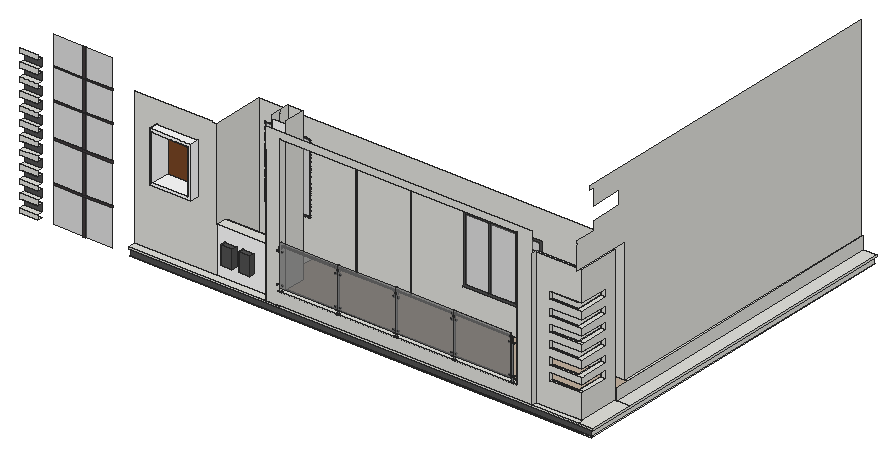
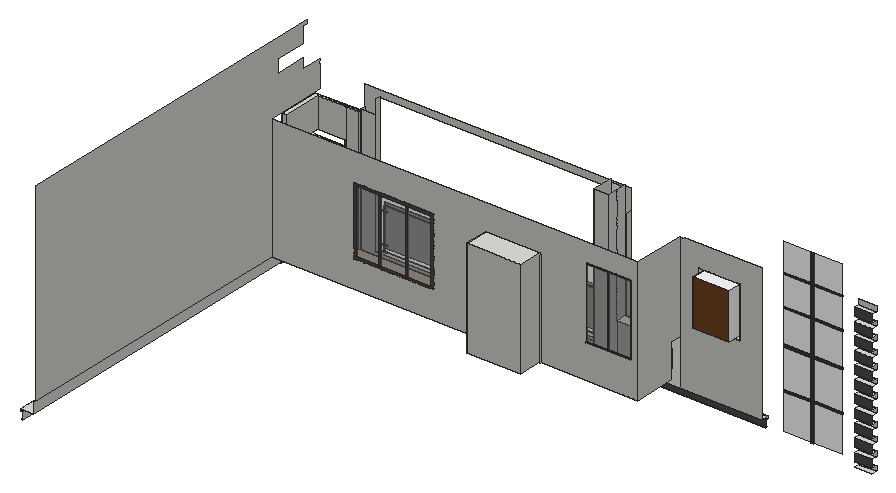
# SketchUp Ruby script. Lengths in inches.
U = 1.inch
M = Sketchup.active_model
def pt(a) = Geom::Point3d.new(a.map { |v| v * U })
def face(e, loops, mat)
  f = e.add_face(loops[0].map { |a| pt(a) })
  loops[1..].each { |l| e.add_face(l.map { |a| pt(a) }).erase! }
  f.material = f.back_material = mat if mat
  f
end
# faces: each face lists its corners as indices into pts; further lists are holes
def faces(e, pts, list, mat = nil) = list.each { |f| face(e, (f[0].is_a?(Array) ? f : [f]).map { |l| l.map { |i| pts[i] } }, mat) }
# xy, xz, yz: faces in a plane at the given z, y or x. An outline is a flat list of corners, or four numbers for a rectangle; further outlines are holes
def ring(l) = l.size == 4 ? [[l[0], l[1]], [l[2], l[1]], [l[2], l[3]], [l[0], l[3]]] : l.each_slice(2).to_a
def flat(e, list, mat, &to3) = list.each { |f| face(e, (f[0].is_a?(Array) ? f : [f]).map { |l| ring(l).map { |u, v| to3.(u, v) } }, mat) }
def xy(e, z, list, mat = nil) = flat(e, list, mat) { |x, y| [x, y, z] }
def xz(e, y, list, mat = nil) = flat(e, list, mat) { |x, z| [x, y, z] }
def yz(e, x, list, mat = nil) = flat(e, list, mat) { |y, z| [x, y, z] }
def lines(e, pts, list) = list.each { |a, b| e.add_line(pt(pts[a]), pt(pts[b])) }
# prism: a flat outline (further loops are holes) pulled along v
def prism(e, loops, v, mat = nil)
  f = face(e, loops, mat); d = Geom::Vector3d.new(v.map { |x| x * U })
  f.pushpull(f.normal.samedirection?(d) ? d.length : -d.length)
end
def box(e, o, s, mat = nil) = prism(e, [[o, [o[0] + s[0], o[1], o[2]], [o[0] + s[0], o[1] + s[1], o[2]], [o[0], o[1] + s[1], o[2]]]], [0, 0, s[2]], mat)
def at(x, y, z, deg = 0) = Geom::Transformation.translation(pt([x, y, z])) * Geom::Transformation.rotation(ORIGIN, Z_AXIS, deg.degrees)
def axes(o, x, y, z) = Geom::Transformation.new([*x, 0, *y, 0, *z, 0, *pt(o).to_a, 1])
def part(name) = M.definitions.add(name)
# library, detail: a bought-in or finely detailed component or shape, given as its bounding box
def library(name, o, s) = part(name).tap { |d| box(d.entities, o, s) }
def detail(e, o, s) = box(e.add_group.entities, o, s)
def put(e, d, t, mat = nil) = e.add_instance(d, t).tap { |i| i.material = mat if mat }
def group(e, t, mat = nil) = e.add_group.tap { |g| g.transformation = t; g.material = mat if mat }.entities
root = M.entities
M.materials.add("[0128_White]").color = [255, 255, 255]
M.materials.add("[0135_DarkGray]").color = [81, 81, 81]
M.materials.add("[Asphalt New]").color = [67, 60, 62]
M.materials.add("[Granite Brown]").color = [113, 117, 119]
M.materials.add("[Granite Light Gray]").color = [139, 143, 145]
M.materials.add("[Stone Brushed Khaki]").color = [166, 166, 164]
M.materials.add("[Tile Large Brown]").color = [195, 178, 159]
M.materials.add("[Translucent Glass Gray]").color = [128, 128, 128]
M.materials["[Translucent Glass Gray]"].alpha = 0.5
M.materials.add("[Wood Veneer 01]").color = [120, 70, 37]
M.materials.add("archibd _ glass railing _ 8mm glass").color = [128, 128, 128]
M.materials["archibd _ glass railing _ 8mm glass"].alpha = 0.5
c1 = part("DOOR12")
g1 = group(c1.entities,at(114.73,28.14,-0.51))
g2 = group(g1,at(0,0,0))
box(g2,[0,0,0],[36,0.5,77.7])
c2 = part("archibd _ glass railing _  tophandrail")
box(c2.entities,[0,0,0],[47.24,2.95,0.98],"[Stone Brushed Khaki]")
c3 = part("archibd _ glass railing _  8 mm Glass")
box(c3.entities,[0.2,-0.31,2.95],[46.85,0.31,44.29],"archibd _ glass railing _ 8mm glass")
p = [[47.05,0,2.95],[47.24,0,2.95],[0.2,0,2.95],[0,0,2.95]]
lines(c3.entities,p,[[0,1],[2,3]])
c4 = part("archibd _ glass railing _  post 1")
box(c4.entities,[-0.04,0,0],[0.47,2.95,41.34],"[Granite Light Gray]")
c5 = part("archibd _ glass railing _ joint plate")
box(c5.entities,[0.98,0.98,-0.31],[2.96,4.93,0.31],"[Granite Light Gray]")
c6 = part("archibd _ glass railing _  post knob")
prism(c6.entities,[[[0.43,1.22,0],[0.43,1.97,0],[0.43,1.97,2.95],[0.43,0,2.95],[0.43,0,0],[0.43,0.75,0],[0.43,0.75,0.98],[0.43,1.22,0.98]]],[-0.47,0,0],"[Granite Light Gray]")
c7 = part("archibd _ glass railing _ serew")
xy(c7.entities,0,[[0.16,0,0,0.27,0.16,0.55,0.47,0.55,0.63,0.27,0.47,0]],"[Granite Brown]")
xy(c7.entities,0.2,[[0.16,0,0.47,0,0.63,0.27,0.47,0.55,0.16,0.55,0,0.27]],"[Granite Brown]")
xz(c7.entities,0,[[0.16,0,0.47,0.2]],"[Granite Brown]")
xz(c7.entities,0.55,[[0.16,0,0.47,0.2]],"[Granite Brown]")
p = [[0,0.27,0],[0.16,0,0],[0.16,0,0.2],[0,0.27,0.2],[0.47,0,0],[0.63,0.27,0],
  [0.63,0.27,0.2],[0.47,0,0.2],[0.16,0.55,0],[0.16,0.55,0.2],[0.47,0.55,0],[0.47,0.55,0.2]]
faces(c7.entities,p,[[0,1,2,3],[4,5,6,7],[8,0,3,9],[5,10,11,6]],"[Granite Brown]")
c8 = part("archibd _ glass railing _  knob 1")
xy(c8.entities,-0.2,[[1.26,-0.47,1.97,-0.24],[1.26,0.08,1.26,2.76,0,2.76,0,3.46,1.97,3.46,1.97,0.08]],"[Granite Light Gray]")
xy(c8.entities,-0.12,[[1.34,-0.24,1.89,0.08]],"[Granite Brown]")
xy(c8.entities,0.43,[[1.34,-0.24,1.89,0.08]],"[Granite Brown]")
xy(c8.entities,0.51,[[1.26,-0.47,1.97,-0.24],[1.26,0.08,1.97,0.08,1.97,3.46,0,3.46,0,2.76,1.26,2.76]],"[Granite Light Gray]")
xz(c8.entities,-0.47,[[1.26,-0.2,1.97,0.51]],"[Granite Light Gray]")
xz(c8.entities,-0.24,[[[1.26,-0.2,1.97,0.51],[1.34,-0.12,1.89,0.43]],[1.34,-0.12,1.89,0.43]],"[Granite Light Gray]")
xz(c8.entities,0.08,[[[1.26,-0.2,1.97,0.51],[1.34,-0.12,1.89,0.43]],[1.34,-0.12,1.89,0.43]],"[Granite Light Gray]")
xz(c8.entities,2.76,[[0,-0.2,1.26,0.51]],"[Granite Light Gray]")
xz(c8.entities,3.46,[[0,-0.2,1.97,0.51]],"[Granite Light Gray]")
yz(c8.entities,0,[[2.76,-0.2,3.46,0.51]],"[Granite Light Gray]")
yz(c8.entities,1.26,[[-0.47,-0.2,-0.24,0.51],[0.08,-0.2,2.76,0.51]],"[Granite Light Gray]")
yz(c8.entities,1.34,[[-0.24,-0.12,0.08,0.43]],"[Granite Brown]")
yz(c8.entities,1.89,[[-0.24,-0.12,0.08,0.43]],"[Granite Brown]")
yz(c8.entities,1.97,[[-0.47,-0.2,-0.24,0.51],[0.08,-0.2,3.46,0.51]],"[Granite Light Gray]")
c9 = part("archibd _ glass railing _  knob 2")
put(c9.entities,c8,at(2.4,0,0))
put(c9.entities,c8,axes([1.93,0,0],[-1,0,0],[0,1,0],[0,0,1]))
c10 = part("archibd _ glass railing _  post")
put(c10.entities,c4,at(1.28,0.98,0.31))
put(c10.entities,c5,at(-0.98,-0.98,0.31))
put(c10.entities,c6,at(0.49,2.66,40.67,-90))
put(c10.entities,c7,at(0.31,4.02,0.31))
put(c10.entities,c7,at(0.31,0.36,0.31))
put(c10.entities,c7,at(2.01,4.02,0.31))
put(c10.entities,c7,at(2.01,0.36,0.31))
put(c10.entities,c9,at(-0.6875,-0.75,6.42))
put(c10.entities,c9,at(-0.6875,-0.65,38.1875))
c11 = part("archibd _ modern glass railing _ 1")
put(c11.entities,c2,at(2.2,2.2,43.62))
put(c11.entities,c3,at(2.2,0.65,0.31))
put(c11.entities,c10,at(0.73,1.22,0))
put(c11.entities,c10,at(47.97,1.22,0))
c12 = part("Archibd+_+Glass+Railing+_+Modern+Glass+Railing+_+1")
put(c12.entities,c11,at(11.52,12.04,0))
put(c12.entities,c11,at(153.25,12.04,0))
put(c12.entities,c11,at(106.01,12.04,0))
put(c12.entities,c11,at(58.76,12.04,0))
xy(root,324.03,[[532.875,578.55,567.67,588.61]])
xy(root,325.125,[[749.43,575.61,1658.1875,575.61,1658.1875,577.48,1630.5625,577.48,1630.5625,578.42,749.43,578.42],[1630.5625,577.48,1658.1875,577.48,1658.1875,1270.99,1655,1270.99,1655,578.42,1630.5625,578.42]])
xy(root,333.75,[[532.875,578.55,567.67,588.61]])
xy(root,338.38,[[749.43,573.8,749.43,578.42,1630.5625,578.42,1630.5625,577.48,1660.625,577.48,1660.625,573.8],[1630.5625,577.48,1660.625,578.42],[1655,578.42,1660.625,1270.99]])
xy(root,341.71,[[1018.16,573.8,1047.4,584.05]])
xy(root,342.73,[[749.43,573.8,1047.4,573.8,1047.4,584.05,1541.95,584.05,1541.95,588.61,749.43,588.61],[1047.4,573.8,1541.95,584.05],[1541.95,573.8,1634.625,583.86],[1634.625,573.8,1660.625,573.8,1660.625,665.53,1631.1875,665.53,1631.1875,583.86,1634.625,583.86],[1634.625,665.53,1660.625,1270.99]])
xy(root,349.59,[[532.875,578.55,567.67,588.61]])
xy(root,359.32,[[532.875,578.55,567.67,588.61]])
xy(root,365.875,[[910.24,610.34,1018.14,691.875],[1633.375,690.6875,1634.625,690.6875,1634.625,1270.99,1630.5,1270.99,1630.5,691.875,1633.375,691.875]])
xy(root,365.875,[[1047.4,588.61,1621.25,588.61,1621.25,665.53,1634.625,665.53,1634.625,690.6875,1633.375,690.6875,1633.375,691.875,1208.65,691.875,1208.65,739.5,1102.33,739.5,1102.33,691.875,1018.14,691.875,1018.14,628.55,1047.4,628.55]],"[Tile Large Brown]")
xy(root,368.26,[[1047.4,573.8,1512.22,584.05]])
xy(root,370.97,[[927.55,577.92,949.64,588.61],[962.05,577.92,984.14,588.61]],"[0135_DarkGray]")
xy(root,375.15,[[532.875,578.55,567.67,588.61]])
xy(root,384.88,[[532.875,578.55,567.67,588.61]])
xy(root,390.46,[[1568.17,583.86,1631.1875,588.61],[1621.25,588.61,1631.1875,642.95]])
xy(root,400.71,[[532.875,578.55,567.67,588.61]])
xy(root,405.06,[[1568.17,583.86,1631.1875,588.61],[1621.25,588.61,1631.1875,642.95]])
xy(root,406.7,[[927.55,577.92,949.64,588.61],[962.05,577.92,984.14,588.61]],"[0135_DarkGray]")
xy(root,410.44,[[532.875,578.55,567.67,588.61]])
xy(root,418.09,[[1568.17,583.86,1631.1875,583.86,1631.1875,642.95,1621.25,642.95,1621.25,588.61,1568.17,588.61]])
xy(root,426.28,[[532.875,578.55,567.67,588.61]])
xy(root,432.68,[[1568.17,583.86,1631.1875,588.61],[1621.25,588.61,1631.1875,642.95]])
xy(root,432.6875,[[910.24,588.61,1018.14,610.34]])
xy(root,436,[[532.875,578.55,567.67,588.61]])
xy(root,447.78,[[1568.17,583.86,1631.1875,583.86,1631.1875,642.95,1621.25,642.95,1621.25,588.61,1568.17,588.61]])
xy(root,451.84,[[532.875,578.55,567.67,588.61]])
xy(root,461.57,[[532.875,578.55,567.67,588.61]])
xy(root,462.37,[[1568.17,583.86,1631.1875,588.61],[1621.25,588.61,1631.1875,642.95]])
xy(root,467.37,[[792.08,571.8,873.44,588.61]],"[0128_White]")
xy(root,472.64,[[797.35,571.8,868.17,609.98]],"[0128_White]")
xy(root,476.09,[[1568.17,583.86,1631.1875,588.61],[1621.25,588.61,1631.1875,642.95]])
xy(root,477.4,[[532.875,578.55,567.67,588.61]])
xy(root,487.13,[[532.875,578.55,567.67,588.61]])
xy(root,490.68,[[1568.17,583.86,1631.1875,588.61],[1621.25,588.61,1631.1875,642.95]])
xy(root,502.96,[[532.875,578.55,567.67,588.61]])
xy(root,504.09,[[1568.17,583.86,1631.1875,583.86,1631.1875,642.95,1621.25,642.95,1621.25,588.61,1568.17,588.61]])
xy(root,512.69,[[532.875,578.55,567.67,588.61]])
xy(root,518.68,[[1568.17,583.86,1631.1875,588.61],[1621.25,588.61,1631.1875,642.95]])
xy(root,528.53,[[532.875,578.55,567.67,588.61]])
xy(root,533.84,[[1568.17,583.86,1621.25,588.61],[1621.25,583.86,1631.1875,642.95]])
xy(root,538.25,[[532.875,578.55,567.67,588.61]])
xy(root,548.43,[[1568.17,583.86,1621.25,588.61],[1621.25,583.86,1631.1875,642.95]])
xy(root,554.09,[[532.875,578.55,567.67,588.61]])
xy(root,558.75,[[1102.33,691.875,1208.65,739.5]])
xy(root,562.02,[[797.35,571.8,868.17,609.98]],"[0128_White]")
xy(root,563.82,[[532.875,578.55,567.67,588.61]])
xy(root,567.29,[[792.08,571.8,873.44,588.61]],"[0128_White]")
xy(root,579.65,[[532.875,578.55,567.67,588.61]])
xy(root,589.38,[[532.875,578.55,567.67,588.61]])
xy(root,605.21,[[532.875,578.55,567.67,588.61]])
xy(root,607.25,[[1541.95,583.86,1631.1875,583.86,1631.1875,665.53,1621.25,665.53,1621.25,588.61,1541.95,588.61]])
xz(root,571.8,[[[792.08,467.37,873.44,567.29],[797.35,472.64,868.17,562.02]]],"[0128_White]")
xz(root,573.8,[[749.43,338.38,1660.625,338.38,1660.625,342.73,1047.4,342.73,1047.4,341.71,1018.16,341.71,1018.16,342.73,749.43,342.73],[1018.16,341.71,1047.4,342.73],[[1018.16,342.73,1541.95,649.875],[1047.4,368.26,1512.22,637.28]]])
xz(root,575.61,[[658.55,327.45,664.15,398.34],[600.1,398.34,658.55,402.19],[658.55,398.34,664.15,402.19],[664.15,398.34,716.99,402.19],[658.55,402.19,664.15,476.93],
  [600.1,476.93,658.55,481.65],[658.55,476.93,664.15,481.65],[664.15,476.93,716.99,481.65],[658.55,481.65,664.15,545.03],[600.1,545.03,658.55,547.98],
  [658.55,545.03,664.15,547.98],[664.15,545.03,716.99,547.98],[658.55,547.98,664.15,605.5],[600.1,605.5,658.55,607.82],[658.55,605.5,664.15,607.82],
  [664.15,605.5,716.99,607.82],[658.55,607.82,664.15,663.68]],"[Asphalt New]")
xz(root,575.61,[[600.1,327.45,658.55,398.34],[664.15,327.45,716.99,398.34],[600.1,402.19,658.55,476.93],[664.15,402.19,716.99,476.93],[600.1,481.65,658.55,545.03],
  [664.15,481.65,716.99,545.03],[600.1,547.98,658.55,605.5],[664.15,547.98,716.99,605.5],[600.1,607.82,658.55,663.68],[664.15,607.82,716.99,663.68]],"[Translucent Glass Gray]")
xz(root,577.92,[[927.55,370.97,949.64,406.7],[962.05,370.97,984.14,406.7]],"[0135_DarkGray]")
xz(root,578.42,[[749.43,325.125,1655,338.38]],"[0135_DarkGray]")
xz(root,578.55,[[532.875,324.03,567.67,333.75],[532.875,349.59,567.67,359.32],[532.875,375.15,567.67,384.88],[532.875,400.71,567.67,410.44],[532.875,426.28,567.67,436],
  [532.875,451.84,567.67,461.57],[532.875,477.4,567.67,487.13],[532.875,502.96,567.67,512.69],[532.875,528.53,567.67,538.25],[532.875,554.09,567.67,563.82],
  [532.875,579.65,567.67,589.38],[532.875,605.21,567.67,614.94]])
xz(root,583.86,[[1541.95,342.73,1631.1875,342.73,1631.1875,390.46,1568.17,390.46,1568.17,405.06,1631.1875,405.06,1631.1875,418.09,1568.17,418.09,1568.17,432.68,1631.1875,432.68,1631.1875,447.78,1568.17,447.78,1568.17,462.37,1631.1875,462.37,1631.1875,476.09,1568.17,476.09,1568.17,490.68,1631.1875,490.68,1631.1875,504.09,1568.17,504.09,1568.17,518.68,1631.1875,518.68,1631.1875,533.84,1568.17,533.84,1568.17,548.43,1631.1875,548.43,1631.1875,607.25,1541.95,607.25]])
xz(root,584.05,[[1018.16,341.71,1018.16,609.09,1047.4,609.09,1047.4,368.26,1512.22,368.26,1512.22,609.09,1541.95,609.09,1541.95,342.73,1047.4,342.73,1047.4,341.71]])
xz(root,588.61,[[[749.43,342.73,910.24,342.73,910.24,602.96,910.19,602.96,910.19,609.09,900.26,609.09,900.26,610.34,753.71,610.34,753.71,610.29,751.95,610.34,749.43,610.34],[792.08,467.37,873.44,567.29]],[1541.95,365.875,1565.61,607.25],[1565.61,365.875,1565.61,607.25,1621.25,607.25,1621.25,548.43,1568.17,548.43,1568.17,533.84,1621.25,533.84,1621.25,518.68,1568.17,518.68,1568.17,504.09,1621.25,504.09,1621.25,490.68,1568.17,490.68,1568.17,476.09,1621.25,476.09,1621.25,462.37,1568.17,462.37,1568.17,447.78,1621.25,447.78,1621.25,432.68,1568.17,432.68,1568.17,418.09,1621.25,418.09,1621.25,405.06,1568.17,405.06,1568.17,390.46,1621.25,390.46,1621.25,365.875],[910.19,602.96,910.24,609.09]])
xz(root,588.61,[[[910.24,342.73,1541.95,342.73,1541.95,365.875,1047.4,365.875,1047.4,656.4,1018.16,656.4,1018.16,662.4375,1018.14,662.4375,1018.14,432.6875,910.24,432.6875],[927.55,370.97,949.64,406.7],[962.05,370.97,984.14,406.7]]],"[0128_White]")
xz(root,588.61,[[532.875,333.75,567.67,349.59],[532.875,359.32,567.67,375.15],[532.875,384.88,567.67,400.71],[532.875,410.44,567.67,426.28],[532.875,436,567.67,451.84],
  [532.875,461.57,567.67,477.4],[532.875,487.13,567.67,502.96],[532.875,512.69,567.67,528.53],[532.875,538.25,567.67,554.09],[532.875,563.82,567.67,579.65],
  [532.875,589.38,567.67,605.21]],"[0135_DarkGray]")
xz(root,609.98,[[797.35,472.64,868.17,562.02]],"[Wood Veneer 01]")
xz(root,610.34,[[910.24,365.875,1018.14,432.6875]])
xz(root,628.55,[[1018.14,365.875,1047.4,662.4375]])
xz(root,642.95,[[1621.25,390.46,1631.1875,405.06],[1621.25,418.09,1631.1875,432.68],[1621.25,447.78,1631.1875,462.37],[1621.25,476.09,1631.1875,490.68],[1621.25,504.09,1631.1875,518.68],
  [1621.25,533.84,1631.1875,548.43]])
xz(root,665.53,[[1631.1875,342.73,1634.625,365.875],[1621.25,365.875,1631.1875,607.25]])
xz(root,691.875,[[[910.24,365.875,1102.33,365.875,1102.33,558.75,1208.65,558.75,1208.65,365.875,1630.5,365.875,1630.5,609.09,910.24,609.09],[1312.03,418.64,1468.72,553.83],[921.72,432.22,1012.47,573.72]]])
xz(root,691.875,[[[1312.03,418.64,1468.72,553.83],[1317.01,423.62,1463.74,548.85]],[1362.03,423.62,1366.35,548.85],[1415.04,423.62,1419.5,548.85]],"[0135_DarkGray]")
xz(root,691.875,[[[921.72,432.22,1012.47,573.72],[923.9,434.4,1010.3,571.55]],[967.1,434.4,969.07,571.55]],"[Asphalt New]")
xz(root,691.875,[[1317.01,423.62,1362.03,548.85],[1366.35,423.62,1415.04,548.85],[1419.5,423.62,1463.74,548.85],[923.9,434.4,967.1,571.55],[969.07,434.4,1010.3,571.55]],"[Translucent Glass Gray]")
xz(root,739.5,[[1102.33,365.875,1208.65,558.75]])
yz(root,792.08,[[571.8,467.37,588.61,567.29]],"[0128_White]")
yz(root,797.35,[[571.8,472.64,609.98,562.02]],"[0128_White]")
yz(root,868.17,[[571.8,472.64,609.98,562.02]],"[0128_White]")
yz(root,873.44,[[571.8,467.37,588.61,567.29]],"[0128_White]")
yz(root,910.24,[[610.34,365.875,691.875,365.875,691.875,609.09,588.61,609.09,588.61,432.6875,610.34,432.6875]])
yz(root,927.55,[[577.92,370.97,588.61,406.7]],"[0135_DarkGray]")
yz(root,949.64,[[577.92,370.97,588.61,406.7]],"[0135_DarkGray]")
yz(root,962.05,[[577.92,370.97,588.61,406.7]],"[0135_DarkGray]")
yz(root,984.14,[[577.92,370.97,588.61,406.7]],"[0135_DarkGray]")
yz(root,1018.14,[[610.34,365.875,628.55,662.4375],[588.61,432.6875,610.34,662.4375]])
yz(root,1018.16,[[573.8,341.71,584.05,609.09]])
yz(root,1047.4,[[573.8,341.71,584.05,342.73],[588.61,365.875,628.55,662.4375],[573.8,368.26,584.05,637.28]])
yz(root,1102.33,[[691.875,365.875,739.5,558.75]])
yz(root,1208.65,[[691.875,365.875,739.5,558.75]])
yz(root,1512.22,[[573.8,368.26,584.05,637.28]])
yz(root,1541.95,[[573.8,342.73,583.86,609.09],[583.86,342.73,584.05,607.25],[584.05,342.73,588.61,607.25],[583.86,607.25,584.05,609.09]])
yz(root,1568.17,[[583.86,390.46,588.61,405.06],[583.86,418.09,588.61,432.68],[583.86,447.78,588.61,462.37],[583.86,476.09,588.61,490.68],[583.86,504.09,588.61,518.68],
  [583.86,533.84,588.61,548.43]])
yz(root,1621.25,[[588.61,365.875,588.61,390.46,642.95,390.46,642.95,393.94,665.53,393.94,665.53,365.875],[642.95,393.94,642.95,405.06,588.61,405.06,588.61,418.09,642.95,418.09,642.95,432.68,588.61,432.68,588.61,447.78,642.95,447.78,642.95,462.37,588.61,462.37,588.61,476.09,642.95,476.09,642.95,490.68,588.61,490.68,588.61,504.09,642.95,504.09,642.95,518.68,588.61,518.68,588.61,533.84,642.95,533.84,642.95,548.43,588.61,548.43,588.61,607.25,665.53,607.25,665.53,393.94]])
yz(root,1630.5,[[691.875,365.875,1270.99,365.875,1270.99,745.125,606.125,745.125,606.125,737.63,613.8125,737.63,613.8125,706.75,676.48,706.75,676.48,681.07,613.8125,681.07,613.8125,662.46,573.8,662.46,573.8,658.77,576.11,658.77,576.11,653.49,573.8,653.49,573.8,609.09,691.875,609.09]])
yz(root,1631.1875,[[583.86,342.73,665.53,342.73,665.53,607.25,583.86,607.25,583.86,548.43,642.95,548.43,642.95,533.84,583.86,533.84,583.86,518.68,642.95,518.68,642.95,504.09,583.86,504.09,583.86,490.68,642.95,490.68,642.95,476.09,583.86,476.09,583.86,462.37,642.95,462.37,642.95,447.78,583.86,447.78,583.86,432.68,642.95,432.68,642.95,418.09,583.86,418.09,583.86,405.06,642.95,405.06,642.95,390.46,583.86,390.46]])
yz(root,1634.625,[[665.53,342.73,1270.99,365.875]])
yz(root,1655,[[578.42,325.125,1270.99,338.38]])
yz(root,1660.625,[[573.8,338.38,1270.99,342.73]])
put(root,c1,axes([758.93,623.4,367.125],[2.98365,0,0],[0,2.44561,0],[0,0,2.44561]))
put(root,c12,axes([1013.44,569.32,367.68],[2.41,0,0],[0,0.3374,0],[0,0,1.8557]))
